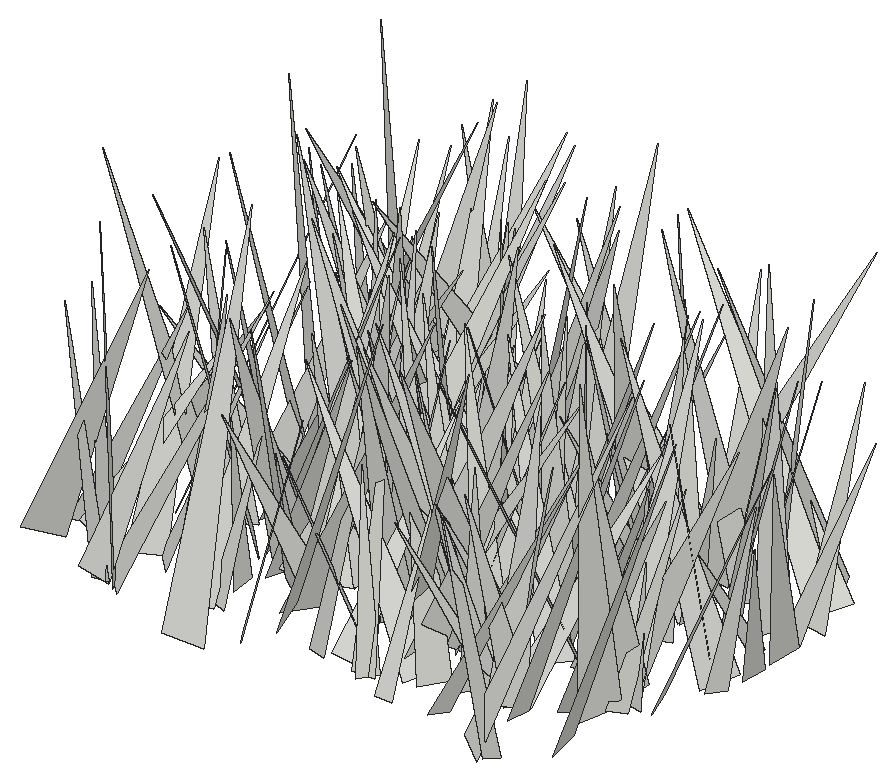
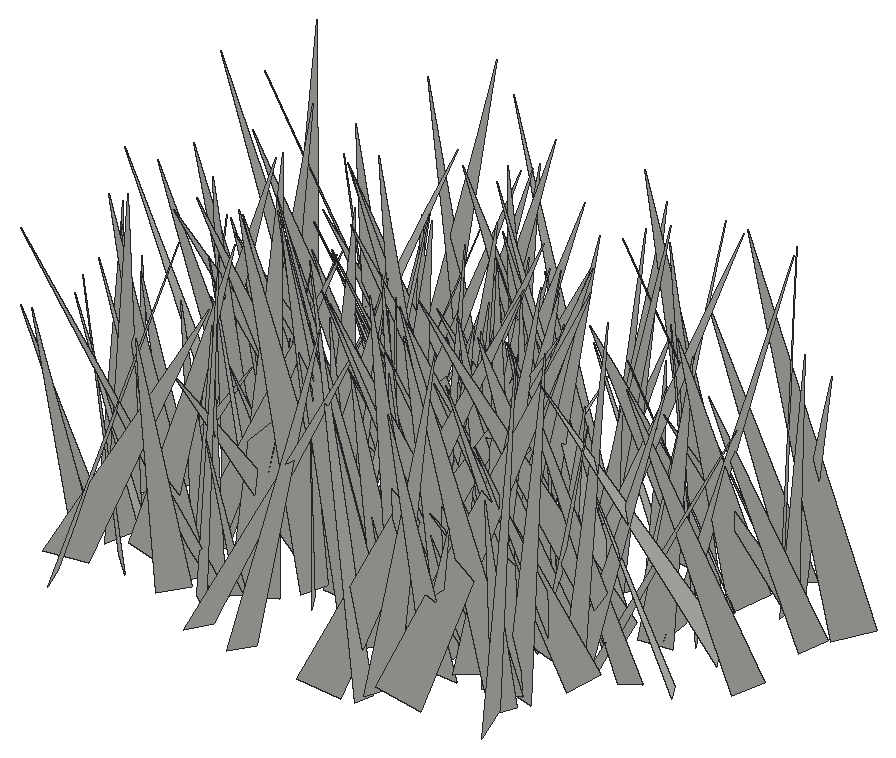
# SketchUp Ruby script. Lengths in inches.
U = 1.inch
M = Sketchup.active_model
def pt(a) = Geom::Point3d.new(a.map { |v| v * U })
def face(e, loops, mat)
  f = e.add_face(loops[0].map { |a| pt(a) })
  loops[1..].each { |l| e.add_face(l.map { |a| pt(a) }).erase! }
  f.material = f.back_material = mat if mat
  f
end
# faces: each face lists its corners as indices into pts; further lists are holes
def faces(e, pts, list, mat = nil) = list.each { |f| face(e, (f[0].is_a?(Array) ? f : [f]).map { |l| l.map { |i| pts[i] } }, mat) }
# xy, xz, yz: faces in a plane at the given z, y or x. An outline is a flat list of corners, or four numbers for a rectangle; further outlines are holes
def ring(l) = l.size == 4 ? [[l[0], l[1]], [l[2], l[1]], [l[2], l[3]], [l[0], l[3]]] : l.each_slice(2).to_a
def flat(e, list, mat, &to3) = list.each { |f| face(e, (f[0].is_a?(Array) ? f : [f]).map { |l| ring(l).map { |u, v| to3.(u, v) } }, mat) }
def xy(e, z, list, mat = nil) = flat(e, list, mat) { |x, y| [x, y, z] }
def xz(e, y, list, mat = nil) = flat(e, list, mat) { |x, z| [x, y, z] }
def yz(e, x, list, mat = nil) = flat(e, list, mat) { |y, z| [x, y, z] }
def lines(e, pts, list) = list.each { |a, b| e.add_line(pt(pts[a]), pt(pts[b])) }
# prism: a flat outline (further loops are holes) pulled along v
def prism(e, loops, v, mat = nil)
  f = face(e, loops, mat); d = Geom::Vector3d.new(v.map { |x| x * U })
  f.pushpull(f.normal.samedirection?(d) ? d.length : -d.length)
end
def box(e, o, s, mat = nil) = prism(e, [[o, [o[0] + s[0], o[1], o[2]], [o[0] + s[0], o[1] + s[1], o[2]], [o[0], o[1] + s[1], o[2]]]], [0, 0, s[2]], mat)
def at(x, y, z, deg = 0) = Geom::Transformation.translation(pt([x, y, z])) * Geom::Transformation.rotation(ORIGIN, Z_AXIS, deg.degrees)
def axes(o, x, y, z) = Geom::Transformation.new([*x, 0, *y, 0, *z, 0, *pt(o).to_a, 1])
def part(name) = M.definitions.add(name)
# library, detail: a bought-in or finely detailed component or shape, given as its bounding box
def library(name, o, s) = part(name).tap { |d| box(d.entities, o, s) }
def detail(e, o, s) = box(e.add_group.entities, o, s)
def put(e, d, t, mat = nil) = e.add_instance(d, t).tap { |i| i.material = mat if mat }
def group(e, t, mat = nil) = e.add_group.tap { |g| g.transformation = t; g.material = mat if mat }.entities
root = M.entities
c1 = part("fur_instance\#9")
p = [[0.8125,0,1.79],[0.67,-0.02,1.48],[0,-0.11,0],[0,0.11,0]]
faces(c1.entities,p,[[0,1,2,3]])
put(root,c1,axes([533.97,55.48,-21.86],[-0.24232,8.0833,1.63068],[8.24361,0.27788,-0.15248],[0.20433,-1.625,8.08549]))
put(root,c1,axes([528.9,56.9,-21.66],[-0.2633,5.21725,2.01289],[5.21535,0.95622,-1.79623],[2.01778,-1.79073,4.90536]))
put(root,c1,axes([529.4,57.44,-21.86],[-5.46878,-3.64969,2.6695],[-4.02035,5.84198,-0.2491],[2.0696,1.70441,6.57007]))
put(root,c1,axes([546.55,55.77,-21.86],[4.64022,6.0526,0.40907],[6.0581,-4.59639,-0.71102],[0.31728,-0.75645,7.59342]))
put(root,c1,axes([525.39,58.47,-21.86],[5.01421,-5.55154,0.43768],[-5.45899,-4.78379,1.86233],[1.10028,1.565,7.24525]))
put(root,c1,axes([529.05,57.08,-21.86],[-2.00481,-4.221,2.16779],[-4.72189,1.54205,-1.3643],[-0.46899,2.51807,4.46932]))
put(root,c1,axes([547.59,55.65,-21.86],[-6.80362,-1.51626,0.05987],[-1.39466,6.13985,-2.9915],[-0.59797,2.93174,6.29597]))
put(root,c1,axes([535.99,58.82,-21.66],[7.97506,1.59703,0.67128],[1.71117,-7.75527,-1.87893],[-0.27022,-1.97686,7.91339]))
put(root,c1,axes([540.6,57.5,-21.86],[-3.29969,1.99263,1.18367],[2.06312,3.46364,-0.07948],[1.05601,-0.54058,3.85386]))
put(root,c1,axes([544.97,59.31,-21.86],[-3.89152,-1.38284,0.09587],[-1.31779,3.77936,1.02238],[0.42995,-0.93252,4.00136]))
put(root,c1,axes([545.88,59.3,-21.86],[3.33283,-3.55166,1.19436],[-3.37517,-3.53973,-1.10774],[-1.62758,0.06765,4.74288]))
put(root,c1,axes([535.45,56.92,-21.86],[3.40494,2.47984,0.75094],[2.39973,-3.48584,0.63038],[-0.97714,0.08048,4.16483]))
put(root,c1,axes([544.68,59.22,-21.86],[-3.58815,0.95471,1.93369],[1.59157,3.70529,1.12394],[1.45517,-1.69849,3.5388]))
put(root,c1,axes([540.6,59.67,-21.86],[7.85727,-0.11013,0.63762],[0.0287,-7.70188,-1.68396],[-0.64642,-1.6806,7.67549]))
put(root,c1,axes([549.01,57.875,-21.86],[7.02887,1.41814,0.69885],[1.44367,-7.05544,-0.2028],[-0.64447,-0.3379,7.16763]))
put(root,c1,axes([542.96,61.66,-21.66],[6.488,-4.94571,0.82766],[-4.48999,-6.33233,-2.64212],[-2.23271,-1.63731,7.71838]))
put(root,c1,axes([542.03,56.59,-21.86],[0.7,4.04155,0.09862],[4.02713,-0.70587,0.34334],[-0.35517,-0.03822,4.08733]))
put(root,c1,axes([529.34,57.43,-21.86],[4.92095,5.18553,0.33695],[5.09859,-4.72846,-1.69263],[1.00379,-1.4039,6.94554]))
put(root,c1,axes([544.14,57.02,-21.86],[5.39304,-0.33096,0.39775],[-0.43435,-5.15892,1.59671],[-0.28121,1.6213,5.16187]))
put(root,c1,axes([540.05,58.48,-21.86],[-3.22375,-2.36609,0.00506],[-2.25529,3.0702,-1.21594],[-0.71558,0.9831,3.80952]))
put(root,c1,axes([544.06,59.04,-21.86],[3.93082,-2.70083,1.38603],[-2.7651,-4.12134,-0.18897],[-1.2529,0.6221,4.76552]))
put(root,c1,axes([531.5,58.91,-21.86],[-0.7765,-5.95979,2.50914],[-6.25232,1.3369,1.24057],[1.65027,2.26084,5.88073]))
put(root,c1,axes([528.24,58.48,-21.86],[-5.05567,-0.39861,1.84756],[-0.46846,5.37567,-0.1221],[1.83109,0.27472,5.06989]))
put(root,c1,axes([540.39,57.51,-21.86],[0.28645,5.00767,1.03913],[5.08565,-0.389,0.47271],[-0.54104,-1.00525,4.99354]))
put(root,c1,axes([545.38,59.42,-21.66],[4.29125,3.34973,1.68987],[3.74545,-3.97458,-1.63261],[-0.21889,-2.33948,5.19327]))
put(root,c1,axes([533.3125,58.22,-21.86],[1.148,3.43718,0.90942],[3.54891,-1.0498,-0.51218],[0.21566,-1.0212,3.58745]))
put(root,c1,axes([542.03,58.66,-21.86],[-4.53112,4.00144,0.54603],[3.94801,4.21612,1.86503],[-0.85024,-1.74745,5.75015]))
put(root,c1,axes([545.71,58.82,-21.86],[3.4619,-5.09824,2.22403],[-5.52391,-3.4582,0.67108],[-0.65172,2.22978,6.12588]))
put(root,c1,axes([548.57,60.4375,-21.86],[6.94101,-3.43299,1.84422],[-3.2352,-7.17632,-1.18245],[-2.17258,-0.28153,7.65277]))
put(root,c1,axes([535.88,60.71,-21.66],[2.95419,-3.46444,1.08183],[-2.95275,-3.10527,-1.88109],[-2.11044,-0.50488,4.14621]))
put(root,c1,axes([534.76,60.64,-21.86],[-2.91514,-5.53327,1.42514],[-5.42873,3.18122,1.24695],[1.78243,0.63944,6.12864]))
put(root,c1,axes([533.13,59.89,-21.86],[3.87563,-0.57439,1.14349],[-0.32332,-3.96837,-0.89752],[-1.23813,-0.76168,3.81378]))
put(root,c1,axes([539.27,61.01,-21.86],[1.68994,-6.65431,0.98946],[-6.7239,-1.70391,0.02495],[-0.21912,0.96522,6.8655]))
put(root,c1,axes([541.9,60.9375,-21.86],[-1.24664,-7.42641,1.30497],[-7.49381,1.07378,-1.04811],[-0.83512,1.45053,7.45702]))
put(root,c1,axes([533.7,62.13,-21.86],[5.49992,-4.64771,0.52674],[-4.40214,-5.41809,-1.84207],[-1.58109,-1.08206,6.96111]))
put(root,c1,axes([544.5,60.12,-21.86],[-7.15146,0.58689,0.88826],[0.71619,7.11549,1.06478],[0.78773,-1.14116,7.09606]))
put(root,c1,axes([544.72,61.21,-21.66],[-4.05266,-1.43323,0.72397],[-1.06557,3.87082,1.69814],[1.20119,-1.40176,3.94899]))
put(root,c1,axes([547.5,61.53,-21.86],[-4.1792,-5.61615,0.15739],[-5.61189,4.16336,-0.45249],[-0.26934,0.3962,6.98585]))
put(root,c1,axes([535.81,59.7,-21.86],[7.07032,-2.50038,0.22823],[-2.5064,-6.98854,1.08245],[0.14815,1.09629,7.42089]))
put(root,c1,axes([539.48,57.69,-21.66],[-1.38897,4.86037,0.26759],[4.61521,1.40338,-1.53442],[1.54748,0.17706,4.81643]))
put(root,c1,axes([535.12,60.7,-21.86],[-3.69542,-5.95234,1.80806],[-6.20183,3.68953,-0.52934],[0.48649,1.82006,6.98615]))
put(root,c1,axes([531.86,62.1875,-21.66],[-4.79038,-5.44103,1.36632],[-5.2062,4.98101,1.5825],[2.08977,-0.06337,7.07448]))
put(root,c1,axes([541.6875,59.07,-21.66],[6.12264,-2.56902,1.18593],[-2.80714,-5.86992,1.77677],[-0.35534,2.10644,6.39763]))
put(root,c1,axes([541.54,62.39,-21.66],[4.33462,-5.23656,1.50263],[-4.77333,-4.57611,-2.17783],[-2.62578,-0.3257,6.43953]))
put(root,c1,axes([546.62,58.33,-21.66],[6.71372,1.26121,1.18447],[0.98901,-6.69183,1.51954],[-1.41968,1.3025,6.66001]))
put(root,c1,axes([538.4,57.41,-21.66],[3.46655,5.88623,0.70358],[5.62008,-3.5225,1.77941],[-1.8861,0.32244,6.59533]))
put(root,c1,axes([548.78,61.95,-21.66],[5.89812,-2.41371,1.85981],[-1.99813,-6.12286,-1.60962],[-2.30052,-0.87028,6.16628]))
put(root,c1,axes([532.94,57.48,-21.66],[-4.70627,4.28235,1.06672],[3.70191,4.67966,-2.45399],[2.40255,1.178,5.87073]))
put(root,c1,axes([538.68,60.09,-21.86],[-2.09497,-3.98677,2.51489],[-4.46346,2.56262,0.34425],[1.51546,2.03632,4.49052]))
put(root,c1,axes([530.01,59.39,-21.86],[3.6626,3.70148,0.35684],[3.71844,-3.64024,-0.40601],[0.03906,-0.53912,5.19141]))
put(root,c1,axes([542.72,58.54,-21.86],[-7.44461,1.33123,0.56849],[1.18187,7.30967,-1.63995],[0.83578,1.52121,7.38274]))
put(root,c1,axes([533.65,61.38,-21.86],[5.62437,-1.82953,0.08499],[-1.8284,-5.62476,-0.0835],[-0.10665,-0.05312,5.91386]))
put(root,c1,axes([526.81,59.31,-21.66],[0.32449,4.79651,0.65441],[4.29347,0.01783,-2.25961],[2.23626,-0.73022,4.24334]))
put(root,c1,axes([525.98,59.98,-21.86],[4.38543,-2.43855,0.87514],[-2.59033,-4.09309,1.5752],[0.05089,1.80126,4.76417]))
put(root,c1,axes([534.14,62.85,-21.86],[-4.63636,-6.55031,0.51962],[-6.56307,4.58532,-0.75728],[-0.32055,0.86066,7.9893]))
put(root,c1,axes([530.36,62.16,-21.86],[-7.66466,-1.90179,1.421],[-1.79066,7.78455,0.75987],[1.55871,-0.40873,7.86043]))
put(root,c1,axes([545.86,59.2,-21.66],[-0.77489,5.32124,0.74593],[4.8544,1.01638,-2.20776],[2.30365,-0.35187,4.90325]))
put(root,c1,axes([539.35,62.51,-21.86],[-0.33805,-5.61743,0.95415],[-5.65981,0.22074,-0.70569],[-0.6576,0.9879,5.58317]))
put(root,c1,axes([539.03,61.74,-21.86],[-2.52237,2.99386,0.77548],[2.99232,2.10973,1.58806],[-0.78138,-1.58517,3.57821]))
put(root,c1,axes([535.83,63.18,-21.66],[2.29516,-7.21123,1.1617],[-7.23425,-2.07612,1.40519],[1.00849,1.5189,7.43607]))
put(root,c1,axes([543.08,61.35,-21.86],[3.04965,-4.5466,3.26672],[-5.09549,-3.79519,-0.52522],[-2.31926,2.35973,5.44941]))
put(root,c1,axes([542.33,61.62,-21.86],[4.26333,-3.02404,0.31767],[-2.97687,-4.03955,1.49732],[0.61963,1.39963,5.00788]))
put(root,c1,axes([546.52,62.2,-21.66],[2.75762,-4.13306,0.47465],[-3.98702,-2.46295,1.71739],[1.18791,1.32801,4.66232]))
put(root,c1,axes([529.37,59.2,-21.66],[-5.90287,3.96424,1.22936],[3.5461,5.92766,-2.08769],[2.15678,1.10365,6.7971]))
put(root,c1,axes([540.08,61.42,-21.66],[4.10846,4.74791,0.21399],[4.46685,-3.7608,-2.31765],[1.62348,-1.66782,5.83529]))
put(root,c1,axes([529.45,62.11,-21.86],[4.80931,3.10321,2.02961],[3.46778,-4.94111,-0.66234],[-1.31293,-1.68352,5.68513]))
put(root,c1,axes([539.33,63.11,-21.86],[-7.26006,2.55391,1.83228],[2.95803,7.11093,1.80912],[1.0629,-2.34529,7.48051]))
put(root,c1,axes([534.35,61.15,-21.66],[0.16131,6.95669,2.04491],[7.08472,0.28432,-1.5261],[1.54396,-2.03146,6.78915]))
put(root,c1,axes([541.75,63.13,-21.86],[-4.06839,-1.50308,0.30492],[-1.46625,4.06536,0.47647],[0.44983,-0.34301,4.31092]))
put(root,c1,axes([541.61,61.125,-21.86],[4.3993,3.63087,0.47155],[3.65139,-4.40515,-0.14642],[-0.27004,-0.41338,5.70225]))
put(root,c1,axes([535.58,61.71,-21.86],[4.7353,0.6555,1.15241],[0.55235,-4.8611,0.49538],[-1.20525,0.34759,4.75472]))
put(root,c1,axes([549.69,62.32,-21.86],[5.84375,1.80801,0.13219],[1.81029,-5.79638,-0.74876],[0.09603,-0.75425,6.07105]))
put(root,c1,axes([532.06,63.14,-21.86],[8.09633,1.85359,0.38508],[1.89305,-7.94545,-1.5559],[-0.02113,-1.6027,8.15877]))
put(root,c1,axes([538.79,62.45,-21.86],[1.17731,-6.81979,2.88625],[-6.91612,0.0321,2.89694],[2.64712,3.11697,6.28517]))
put(root,c1,axes([548.91,60.95,-21.86],[3.7026,-0.58317,1.91769],[-1.4169,-3.61072,1.63767],[-1.41775,2.08554,3.37155]))
put(root,c1,axes([537.01,63.67,-21.86],[-5.38028,-3.08502,1.66928],[-3.07413,5.61908,0.47644],[1.68926,0.39986,6.18367]))
put(root,c1,axes([549.27,61.52,-21.86],[1.77865,4.09096,1.0407],[3.89915,-2.02489,1.29578],[-1.61729,-0.38272,4.26855]))
put(root,c1,axes([538.27,61.4,-21.86],[3.62964,3.56201,0.97293],[3.43547,-3.75775,0.94107],[-1.35352,0.01415,4.99765]))
put(root,c1,axes([530.37,63.27,-21.86],[1.39978,-5.30319,2.32473],[-5.64349,-1.78474,-0.67328],[-1.29585,2.04412,5.44334]))
put(root,c1,axes([545.08,62.35,-21.86],[-3.19469,4.99874,1.10839],[5.10889,3.02549,1.08057],[-0.33936,-1.5103,5.83317]))
put(root,c1,axes([547.44,63.49,-21.86],[1.83372,-5.8574,1.52699],[-5.60076,-1.03656,2.74963],[2.29617,2.14936,5.48737]))
put(root,c1,axes([536.4,66.05,-21.86],[-0.43827,-6.52973,0.002],[-6.42899,0.43186,1.145],[1.14256,-0.07472,6.44348]))
put(root,c1,axes([525.88,63.71,-21.86],[3.57334,-4.4658,0.19156],[-4.12422,-3.19939,2.34597],[1.72363,1.60293,5.21618]))
put(root,c1,axes([538.46,61.96,-21.86],[-6.04879,4.39479,0.23194],[4.40071,6.03643,0.38865],[-0.04117,-0.45072,7.46666]))
put(root,c1,axes([536.81,64.84,-21.86],[1.52104,-3.59534,0.18519],[-3.58042,-1.53172,-0.32978],[-0.37596,0.04131,3.88989]))
put(root,c1,axes([536.49,63,-21.86],[-8.05212,1.79962,1.36323],[1.82873,8.16018,0.02927],[1.32393,-0.32629,8.25072]))
put(root,c1,axes([548.24,61.95,-21.86],[-1.91497,6.86191,1.78883],[6.91485,2.21764,-1.10438],[1.57179,-1.39609,7.03799]))
put(root,c1,axes([538.52,61.39,-21.86],[-5.7713,0.32455,0.04644],[0.28097,5.31808,-2.2482],[0.16895,2.24233,5.3253]))
put(root,c1,axes([547.52,59.8,-21.86],[6.83312,3.40706,1.30672],[2.45514,-6.34476,3.70451],[-2.69961,2.8536,6.67654]))
put(root,c1,axes([530.91,65.98,-21.86],[-4.92347,-1.39259,0.14711],[-1.23579,4.5738,1.93769],[0.65861,-1.82825,4.73553]))
put(root,c1,axes([540.01,63.07,-21.86],[-5.43325,1.77797,0.85582],[1.73658,5.49897,-0.39929],[0.93695,0.1182,5.7028]))
put(root,c1,axes([550.41,64.81,-21.86],[-6.07802,2.92755,1.98205],[3.37511,5.97833,1.51972],[1.05246,-2.26504,6.57292]))
put(root,c1,axes([536.82,62.57,-21.66],[-6.72767,0.28008,1.7782],[-0.11729,6.79671,-1.51427],[1.7963,1.49276,6.56102]))
put(root,c1,axes([543.37,64.81,-21.86],[-3.30956,4.62511,3.28339],[5.43338,3.67626,0.29816],[1.62808,-2.86687,5.67942]))
put(root,c1,axes([538.91,65.07,-21.86],[-1.94061,6.26278,4.61542],[7.19839,3.24975,-1.38302],[2.95087,-3.80883,6.40903]))
put(root,c1,axes([541.08,66.8,-21.66],[-4.09949,-5.26965,1.04192],[-4.89422,4.20438,2.00758],[2.21389,-0.46331,6.36747]))
put(root,c1,axes([536.6,64.3125,-21.86],[0.81184,5.62301,2.88886],[5.96448,-1.64652,1.52868],[-2.09495,-2.50871,5.47179]))
put(root,c1,axes([550.75,64.2,-21.86],[3.49135,-1.63355,1.08284],[-1.80913,-3.53699,0.49727],[-0.7537,0.9229,3.8224]))
put(root,c1,axes([551.04,65.91,-21.86],[3.9114,-1.46291,0.01114],[-1.40736,-3.77134,-1.11157],[-0.39945,-1.03737,4.02536]))
put(root,c1,axes([537.81,62.34,-21.66],[-6.09704,1.94582,1.05535],[1.61207,6.02238,-1.79053],[1.51697,1.42075,6.14444]))
put(root,c1,axes([532.88,65.65,-21.86],[2.96444,-3.24193,0.90441],[-3.19075,-3.09049,-0.61962],[-1.07107,0.23387,4.34903]))
put(root,c1,axes([540.35,66.03,-21.86],[-7.32197,2.2534,1.35544],[2.57225,6.97064,2.30649],[0.54639,-2.61889,7.30542]))
put(root,c1,axes([544.87,62.71,-21.66],[6.92746,0.46404,1.30725],[0.06508,-6.75935,2.05449],[-1.38564,2.00246,6.63205]))
put(root,c1,axes([546.35,67.28,-21.86],[-5.03232,-2.4099,0.87584],[-1.92345,4.82363,2.22078],[1.6956,-1.68045,5.11859]))
put(root,c1,axes([548.48,66.56,-21.86],[-3.5454,-4.09399,1.47684],[-3.82101,3.83994,1.47185],[2.08366,0.07566,5.21193]))
put(root,c1,axes([537.85,66.05,-21.86],[3.71105,4.69804,3.51461],[5.68502,-3.90755,-0.77947],[-1.45074,-3.29476,5.93598]))
put(root,c1,axes([531.3,64.33,-21.86],[4.45979,0.0367,0.09292],[0.01604,-4.35825,0.95137],[-0.0986,0.95079,4.35729]))
put(root,c1,axes([533.35,65,-21.86],[2.46567,3.17158,1.58955],[3.37143,-2.69731,0.15219],[-1.10413,-1.15357,4.01439]))
put(root,c1,axes([546.66,65.7,-21.86],[3.53738,-5.32848,1.99163],[-5.66565,-3.51029,0.67133],[-0.50966,2.039,6.36044]))
put(root,c1,axes([535.91,63.09,-21.66],[0.28527,8.21503,1.11931],[7.94931,0.04717,-2.37217],[2.35543,-1.15413,7.87026]))
put(root,c1,axes([542.47,65.17,-21.86],[6.68807,0.43229,0.66728],[0.41432,-6.71942,0.20043],[-0.67859,0.15798,6.69903]))
put(root,c1,axes([536.4,66.79,-21.66],[1.94153,-7.03493,2.68991],[-6.84514,-2.80689,-2.40016],[-3.14163,1.7682,6.89195]))
put(root,c1,axes([535.51,61.82,-21.86],[-6.01479,5.28528,0.0687],[5.03484,5.76049,-2.36301],[1.60915,1.73181,7.65037]))
put(root,c1,axes([535.76,68.4375,-21.86],[5.51839,-2.97407,0.09463],[-2.75984,-5.19025,-2.17974],[-1.11235,-1.87694,5.87762]))
put(root,c1,axes([536.02,65.14,-21.86],[0.77097,6.55392,2.92574],[6.60675,-1.79779,2.28627],[-2.8044,-2.43357,6.19042]))
put(root,c1,axes([551,67.65,-21.86],[5.13341,-1.95182,0.40555],[-1.78394,-4.9977,-1.47188],[-0.88973,-1.24068,5.29103]))
put(root,c1,axes([538.32,65.2,-21.86],[4.52049,-0.19473,1.20973],[-0.39564,-4.60837,0.73662],[-1.15967,0.81315,4.46432]))
put(root,c1,axes([528.23,62.38,-21.66],[6.17595,4.1917,0.11311],[3.92557,-5.85042,2.46738],[-1.47413,1.98185,7.04448]))
put(root,c1,axes([537.85,64.15,-21.86],[-1.08496,4.24211,0.2137],[4.12597,1.10497,-0.98676],[1.00871,0.04308,4.26602]))
put(root,c1,axes([527.76,65.52,-21.86],[3.83341,2.26597,0.28943],[2.28132,-3.82668,-0.25597],[-0.11822,-0.36786,4.44568]))
put(root,c1,axes([531.36,66.17,-21.86],[-3.64938,-5.29226,1.74557],[-5.55344,3.28039,-1.66476],[-0.463,2.36729,6.20923]))
put(root,c1,axes([532.6,65.26,-21.66],[4.39475,-2.24157,1.41228],[-2.61052,-4.13054,1.56743],[-0.4521,2.06082,4.67778]))
put(root,c1,axes([536.87,66.63,-21.86],[5.44749,2.02001,0.26599],[2.02291,-5.27178,-1.39377],[0.24298,-1.39796,5.64031]))
put(root,c1,axes([542.34,65.46,-21.86],[0.9151,5.15761,1.58711],[5.35443,-1.06795,0.38322],[-0.67079,-1.48856,5.22413]))
put(root,c1,axes([544.92,67.34,-21.86],[3.69815,0.46024,1.83595],[1.02421,-3.87534,-1.09159],[-1.5917,-1.42435,3.56322]))
put(root,c1,axes([529.3,65.98,-21.86],[1.94999,6.06367,1.85826],[6.06829,-1.21894,-2.39034],[1.84311,-2.40204,5.90397]))
put(root,c1,axes([543,66.3,-21.66],[1.40362,-5.52471,3.15038],[-5.88186,-2.35471,-1.50878],[-2.41887,2.51999,5.49692]))
put(root,c1,axes([534.74,65.8,-21.86],[-2.8521,5.31504,2.52319],[5.50682,3.39878,-0.93481],[2.07151,-1.71732,5.95905]))
put(root,c1,axes([550.04,67.32,-21.86],[-0.53868,-3.7535,0.51973],[-3.36849,0.23389,-1.80211],[-1.73555,0.71104,3.33637]))
put(root,c1,axes([543.4,65.91,-21.86],[3.9948,0.59542,0.26899],[0.55235,-3.96784,0.58004],[-0.34899,0.53573,3.99706]))
put(root,c1,axes([544.72,67.75,-21.86],[-4.88015,-2.78524,1.52655],[-2.68194,5.11285,0.7548],[1.7015,0.07051,5.5681]))
put(root,c1,axes([546.41,65.5,-21.86],[4.62309,3.63215,1.82021],[3.50208,-4.96051,1.00367],[-2.05939,-0.28182,5.79293]))
put(root,c1,axes([539.7,66.9,-21.86],[-6.42815,4.45601,0.04956],[4.21627,6.0534,2.59983],[-1.44275,-2.16333,7.37686]))
put(root,c1,axes([543.35,69.28,-21.86],[4.3126,-6.65441,0.44802],[-6.65528,-4.32849,-0.22777],[-0.435,0.25174,7.9264]))
put(root,c1,axes([533.91,64.76,-21.66],[-6.55777,-1.69063,0.96933],[-1.94723,5.82112,-3.02077],[0.07829,3.17151,6.06115]))
put(root,c1,axes([531.67,66.08,-21.66],[3.01287,6.59159,3.14785],[6.68601,-3.85992,1.68335],[-2.94198,-2.02171,7.04931]))
put(root,c1,axes([531.13,64,-21.66],[8.13391,1.72844,0.70897],[1.41113,-7.75982,2.72846],[-1.22428,2.53935,7.85515]))
put(root,c1,axes([534.82,65.23,-21.66],[4.52009,6.67395,0.30614],[6.59904,-4.40227,-1.46264],[1.04307,-1.07006,7.92676]))
put(root,c1,axes([539.6,66.36,-21.86],[-5.47988,-2.79163,2.54101],[-3.31815,5.69792,-0.89593],[1.79996,2.00489,6.08438]))
put(root,c1,axes([546.87,67.69,-21.86],[4.24921,-1.39082,0.67887],[-1.35455,-4.30166,-0.33452],[-0.74864,-0.11098,4.4585]))
put(root,c1,axes([532.31,69.36,-21.66],[1.32188,-7.44707,0.58602],[-7.30684,-1.16527,1.67389],[1.55318,0.85612,7.37593]))
put(root,c1,axes([548.48,67.73,-21.86],[5.73568,-0.06882,1.05766],[0.01363,-5.81521,-0.45231],[-1.05981,-0.44725,5.71823]))
put(root,c1,axes([530.59,66.96,-21.86],[4.87522,-3.55324,0.35007],[-3.38958,-4.41978,2.34354],[1.12198,2.08707,5.55888]))
put(root,c1,axes([546.73,68.17,-21.86],[-6.88709,2.46248,0.81316],[2.58785,6.67518,1.70354],[0.16756,-1.88022,7.11293]))
put(root,c1,axes([533.78,69.11,-21.66],[-6.33507,2.2676,3.27677],[3.13305,6.63723,1.4641],[2.46237,-2.61105,6.56746]))
put(root,c1,axes([533.55,65.67,-21.86],[3.64416,1.65962,0.06909],[1.4569,-3.27351,1.789],[-0.79783,1.60274,3.58241]))
put(root,c1,axes([538.33,67.8,-21.66],[4.58596,6.39713,1.96066],[6.63658,-4.04695,-2.31874],[0.85046,-2.91504,7.52182]))
put(root,c1,axes([541.5,68.37,-21.86],[4.52719,2.71843,2.25301],[3.1828,-4.72799,-0.69084],[-1.52829,-1.79378,5.23527]))
put(root,c1,axes([548.59,67.32,-21.86],[4.95919,2.18923,1.00137],[2.21006,-5.04934,0.09393],[-0.95452,-0.31696,5.4201]))
put(root,c1,axes([531.69,66.39,-21.66],[4.95008,1.27612,1.12304],[0.89586,-4.89693,1.61571],[-1.4447,1.33589,4.84988]))
put(root,c1,axes([541.05,67.43,-21.86],[1.36969,7.27883,2.41401],[7.66649,-1.2409,-0.6083],[0.18385,-2.48268,7.38156]))
put(root,c1,axes([535.22,68.45,-21.86],[4.24569,0.44069,0.96407],[0.53821,-4.32495,-0.39327],[-0.91322,-0.50013,4.25034]))
put(root,c1,axes([538.9,67.32,-21.86],[3.58302,-2.92408,2.58959],[-3.63927,-3.77537,0.77237],[-1.41842,2.30013,4.5598]))
put(root,c1,axes([531.73,69.14,-21.86],[1.75829,5.41715,3.42251],[6.36736,-1.87488,-0.30363],[-0.71818,-3.36006,5.68726]))
put(root,c1,axes([533.38,67.57,-21.86],[2.97178,5.39968,0.42783],[5.06638,-2.59832,-2.39825],[1.91609,-1.5044,5.67771]))
put(root,c1,axes([538.81,68.4,-21.86],[4.56446,-0.76979,0.5853],[-0.81155,-4.58493,0.29877],[-0.52586,0.39409,4.61927]))
put(root,c1,axes([538.04,69.66,-21.86],[4.04324,-6.81137,0.9787],[-6.74817,-3.70246,2.11055],[1.34718,1.89668,7.63467]))
put(root,c1,axes([543.45,65.85,-21.86],[5.35308,0.77922,1.1136],[0.09871,-4.73607,2.83947],[-1.35556,2.73224,4.60435]))
put(root,c1,axes([533.17,66.16,-21.86],[1.53253,6.73152,0.42824],[6.72346,-1.5597,0.45586],[-0.5402,-0.31526,6.8887]))
put(root,c1,axes([535.23,70.74,-21.86],[7.23074,-0.77372,0.74856],[-0.57311,-7.06946,-1.77111],[-0.91134,-1.69312,7.05304]))
put(root,c1,axes([534.71,72.12,-21.66],[1.87232,-8.06563,0.81969],[-7.60481,-2.03883,-2.69107],[-2.80947,0.14362,7.83059]))
put(root,c1,axes([545.71,70.04,-21.66],[2.64878,-6.42579,1.07864],[-6.29914,-2.22772,2.19734],[1.66585,1.79353,6.59382]))
put(root,c1,axes([549.59,68.79,-21.86],[6.19428,-1.57461,3.33029],[-1.87234,-6.95675,0.19327],[-3.17247,1.03131,6.38836]))
put(root,c1,axes([541.68,67.46,-21.66],[6.54564,-3.57049,3.76512],[-4.66006,-6.71077,1.73761],[-2.28219,3.46223,7.25083]))
put(root,c1,axes([537.33,73.26,-21.66],[4.76692,-6.38187,0.99404],[-5.33821,-4.5884,-3.85875],[-3.63592,-1.6304,6.96863]))
put(root,c1,axes([550.375,68.89,-21.86],[1.81296,4.05322,0.9149],[4.0683,-1.5284,-1.29051],[0.84535,-1.3371,4.24853]))
put(root,c1,axes([548.53,68.78,-21.86],[4.35259,2.65064,0.87547],[2.69973,-4.40951,-0.0717],[-0.70982,-0.51745,5.09567]))
put(root,c1,axes([547.96,69.56,-21.66],[-0.65544,-6.57541,2.82853],[-6.91722,-0.14862,-1.94837],[-1.84083,2.89967,6.31422]))
put(root,c1,axes([543.96,70.44,-21.86],[-3.79405,-1.81524,0.00607],[-1.81515,3.79397,0.03081],[0.01877,-0.02517,4.20582]))
put(root,c1,axes([545.43,69.25,-21.86],[-1.15441,5.11883,1.74969],[5.40957,1.09949,0.35248],[0.0216,-1.78472,5.23554]))
put(root,c1,axes([533.13,67.85,-21.86],[-0.22471,7.89617,1.63504],[7.5306,0.79034,-2.78188],[2.88322,-1.44886,7.39332]))
put(root,c1,axes([534.1,68.43,-21.66],[3.571,6.90444,0.98118],[6.89309,-3.32732,-1.67343],[1.05801,-1.62595,7.59098]))
put(root,c1,axes([535.32,67.83,-21.66],[5.43527,-3.00495,4.38513],[-4.48513,-5.95873,1.47596],[-2.85354,3.64214,6.0327]))
put(root,c1,axes([535.43,70.32,-21.86],[1.79677,-5.19077,1.98742],[-5.55817,-1.66844,0.66734],[0.02536,2.09632,5.45226]))
put(root,c1,axes([537.04,68.56,-21.86],[-0.16365,8.04006,1.71484],[8.20749,0.06185,0.49328],[-0.46944,-1.72152,8.02659]))
put(root,c1,axes([532.07,69.55,-21.66],[0.54119,7.40359,2.44886],[7.61955,0.0202,-1.74498],[1.65906,-2.50787,7.21533]))
put(root,c1,axes([543.86,69.4,-21.86],[1.21689,3.56799,0.58582],[3.55761,-1.29191,0.47847],[-0.64586,-0.39367,3.73931]))
put(root,c1,axes([535.29,69.98,-21.86],[-2.90723,2.3787,0.42473],[2.40963,2.90345,0.23285],[0.1797,-0.4498,3.74913]))
put(root,c1,axes([550.57,69.77,-21.86],[0.17579,4.7582,1.26729],[4.89735,-0.03702,-0.54033],[0.51227,-1.27889,4.73069]))
put(root,c1,axes([531.51,70.23,-21.86],[-3.40994,2.09099,1.78678],[2.1335,3.80705,-0.3836],[1.73581,-0.57158,3.98156]))
put(root,c1,axes([544.43,70.92,-21.86],[-4.17203,-5.0841,2.64194],[-5.48144,4.49304,-0.00972],[1.66784,2.04897,6.57676]))
put(root,c1,axes([535.85,72.6,-21.86],[7.53646,1.85279,1.2332],[2.16443,-7.11553,-2.53698],[-0.51849,-2.77277,7.33449]))
put(root,c1,axes([548.39,70.39,-21.86],[3.88828,4.27161,1.82836],[4.44707,-4.1121,0.14976],[-1.3465,-1.2459,5.77433]))
put(root,c1,axes([543.54,72.17,-21.86],[-6.98354,0.71492,0.27676],[0.75932,6.7998,1.59491],[0.10557,-1.6153,6.83646]))
put(root,c1,axes([549.64,72.67,-21.86],[-6.20771,-3.16783,0.82777],[-3.08728,6.25411,0.78157],[1.09042,-0.32718,6.92531]))
put(root,c1,axes([541.44,72.41,-21.86],[-6.05597,0.77226,2.0179],[1.21073,6.18666,1.26588],[1.78953,-1.57224,5.97233]))
put(root,c1,axes([544.51,69.83,-21.86],[3.82071,6.83533,0.31448],[6.59967,-3.58608,-2.23672],[1.80694,-1.35528,7.50444]))
put(root,c1,axes([535.74,71.78,-21.86],[-6.59669,1.20746,2.1658],[1.44471,6.87425,0.5679],[2.0153,-0.97558,6.6822]))
put(root,c1,axes([534.84,69.64,-21.86],[-0.26987,6.47949,0.83868],[6.52839,0.23411,0.29205],[-0.25936,-0.84936,6.47853]))
put(root,c1,axes([531.31,71.22,-21.86],[-7.32615,-2.19993,2.60741],[-2.57876,7.61493,-0.82074],[2.23345,1.57604,7.60517]))
put(root,c1,axes([550.26,71.16,-21.86],[-5.28258,5.45364,0.12335],[5.18528,4.96674,2.47132],[-1.69419,-1.80343,7.17917]))
put(root,c1,axes([545.88,70.65,-21.86],[3.74309,-3.05687,3.19875],[-4.02453,-4.09315,0.7978],[-1.83838,2.73658,4.76642]))
